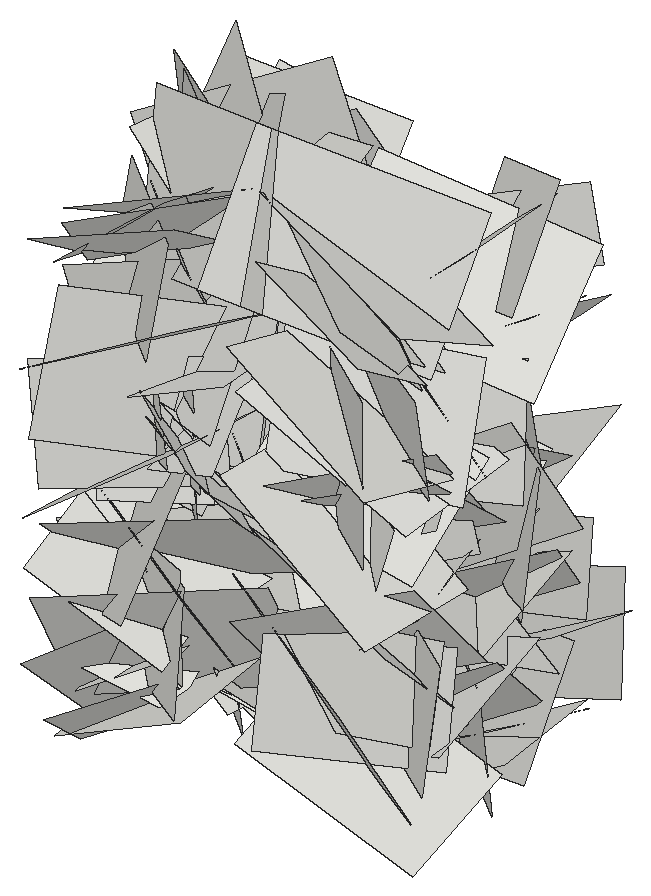
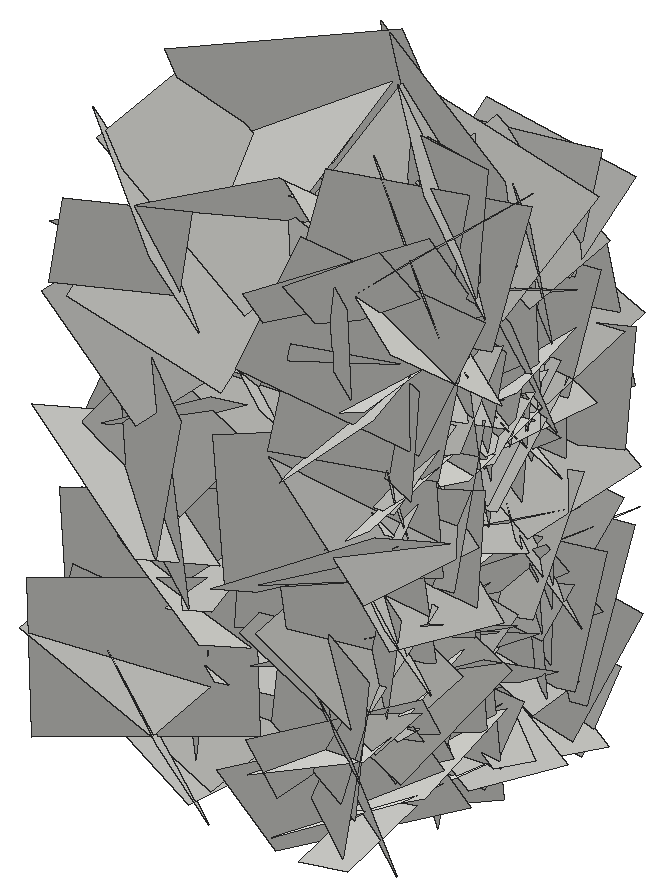
# SketchUp Ruby script. Lengths in inches.
U = 1.inch
M = Sketchup.active_model
def pt(a) = Geom::Point3d.new(a.map { |v| v * U })
def face(e, loops, mat)
  f = e.add_face(loops[0].map { |a| pt(a) })
  loops[1..].each { |l| e.add_face(l.map { |a| pt(a) }).erase! }
  f.material = f.back_material = mat if mat
  f
end
# faces: each face lists its corners as indices into pts; further lists are holes
def faces(e, pts, list, mat = nil) = list.each { |f| face(e, (f[0].is_a?(Array) ? f : [f]).map { |l| l.map { |i| pts[i] } }, mat) }
# xy, xz, yz: faces in a plane at the given z, y or x. An outline is a flat list of corners, or four numbers for a rectangle; further outlines are holes
def ring(l) = l.size == 4 ? [[l[0], l[1]], [l[2], l[1]], [l[2], l[3]], [l[0], l[3]]] : l.each_slice(2).to_a
def flat(e, list, mat, &to3) = list.each { |f| face(e, (f[0].is_a?(Array) ? f : [f]).map { |l| ring(l).map { |u, v| to3.(u, v) } }, mat) }
def xy(e, z, list, mat = nil) = flat(e, list, mat) { |x, y| [x, y, z] }
def xz(e, y, list, mat = nil) = flat(e, list, mat) { |x, z| [x, y, z] }
def yz(e, x, list, mat = nil) = flat(e, list, mat) { |y, z| [x, y, z] }
def lines(e, pts, list) = list.each { |a, b| e.add_line(pt(pts[a]), pt(pts[b])) }
# prism: a flat outline (further loops are holes) pulled along v
def prism(e, loops, v, mat = nil)
  f = face(e, loops, mat); d = Geom::Vector3d.new(v.map { |x| x * U })
  f.pushpull(f.normal.samedirection?(d) ? d.length : -d.length)
end
def box(e, o, s, mat = nil) = prism(e, [[o, [o[0] + s[0], o[1], o[2]], [o[0] + s[0], o[1] + s[1], o[2]], [o[0], o[1] + s[1], o[2]]]], [0, 0, s[2]], mat)
def at(x, y, z, deg = 0) = Geom::Transformation.translation(pt([x, y, z])) * Geom::Transformation.rotation(ORIGIN, Z_AXIS, deg.degrees)
def axes(o, x, y, z) = Geom::Transformation.new([*x, 0, *y, 0, *z, 0, *pt(o).to_a, 1])
def part(name) = M.definitions.add(name)
# library, detail: a bought-in or finely detailed component or shape, given as its bounding box
def library(name, o, s) = part(name).tap { |d| box(d.entities, o, s) }
def detail(e, o, s) = box(e.add_group.entities, o, s)
def put(e, d, t, mat = nil) = e.add_instance(d, t).tap { |i| i.material = mat if mat }
def group(e, t, mat = nil) = e.add_group.tap { |g| g.transformation = t; g.material = mat if mat }.entities
root = M.entities
c1 = part("Component\#6")
p = [[0.01,0,0],[0,3.24,4.54],[4.32,3.24,4.54],[4.33,0,0]]
faces(c1.entities,p,[[0,1,2,3]])
put(root,c1,axes([24.34,147.32,10.4375],[-0.06119,-0.47987,-0.75245],[-0.01649,-0.75336,0.48165],[0.94584,-0.04418,-0.04028]))
put(root,c1,axes([28.31,136.7,5.12],[-0.11008,0.58852,-0.4619],[0.03608,-0.46213,-0.59646],[-0.7922,-0.10282,0.03702]))
put(root,c1,axes([28.31,135.6875,17.375],[0.11773,0.10526,0.9962],[0.108,0.99592,-0.11659],[-1.05635,0.11356,0.09911]))
put(root,c1,axes([28.31,144.39,10.35],[0.12238,0.87118,-0.30871],[0.00416,-0.31157,-0.87778],[-0.97971,0.1075,-0.04229]))
put(root,c1,axes([24.34,139.94,18.75],[-0.02341,-0.9115,0.17831],[-0.09444,0.17962,0.90714],[0.97996,-0.00447,0.09169]))
put(root,c1,axes([28.31,141.47,13.3125],[0.15098,-0.93805,0.13539],[0.00567,0.13771,0.94846],[-1.00463,-0.1402,0.0257]))
put(root,c1,axes([28.31,143.17,8.1],[-0.04482,0.75985,0.07181],[-0.00358,0.07173,-0.76102],[-0.80902,-0.04241,-0.00061]))
put(root,c1,axes([28.31,139.62,7.21],[0.15609,-0.9187,-0.23757],[0.00588,-0.23958,0.92989],[-1.00583,-0.14396,-0.03143]))
put(root,c1,axes([24.34,145.65,3.28],[0.1646,0.60158,-0.34623],[0.0091,-0.35642,-0.61544],[0.73568,-0.13018,0.08507]))
put(root,c1,axes([28.31,141.35,5.69],[-0.05421,0.52298,-0.48745],[-0.04158,-0.49001,-0.52162],[-0.75668,-0.01054,0.06359]))
put(root,c1,axes([24.34,143.03,2.65],[-0.18528,-0.93043,-0.12384],[0.14778,-0.15031,0.9325],[0.98392,-0.15263,-0.16338]))
put(root,c1,axes([28.31,149.3125,5.88],[0.15882,-0.57412,-0.80425],[0.08368,-0.80389,0.58857],[-1.04409,-0.15176,-0.07517]))
put(root,c1,axes([28.31,141.5625,11.54],[0.13399,-0.80117,0.38482],[-0.02481,0.38556,0.81039],[-0.9418,-0.12414,0.0334]))
put(root,c1,axes([28.31,147.06,19.23],[0.16196,0.05609,-0.92604],[-0.00217,-0.93849,-0.05718],[-0.9834,0.01131,-0.15239]))
put(root,c1,axes([24.34,141.85,18.04],[-0.12661,-0.3078,1.12748],[-0.24587,1.11705,0.28038],[1.21422,0.1941,0.17434]))
put(root,c1,axes([28.31,142.57,12.97],[0.12959,-0.66136,0.5647],[-0.03976,0.56572,0.67067],[-0.92097,-0.11748,0.0505]))
put(root,c1,axes([28.31,147.56,10.64],[-0.00206,-0.13591,-0.77504],[0.03252,-0.77447,0.13573],[-0.83344,-0.02988,0.00721]))
put(root,c1,axes([24.34,143.95,11.7],[-0.02215,-0.88691,-0.38082],[-0.08723,-0.37788,0.88459],[1.0194,-0.05161,0.06742]))
put(root,c1,axes([24.34,144.05,16.5],[0.02895,-0.76847,-0.41691],[-0.01722,-0.41749,0.76847],[0.92657,0.01625,0.02731]))
put(root,c1,axes([28.31,143.33,2.25],[-0.06381,-0.71847,0.0034],[0.02834,0.00117,0.7205],[-0.76106,0.06028,0.02655]))
put(root,c1,axes([24.34,147.01,9.44],[-0.18802,-1.10018,-0.17062],[-0.06994,-0.16208,1.11371],[1.17806,-0.18521,0.03889]))
put(root,c1,axes([24.34,143.66,16.18],[0.1105,0.58717,-0.52568],[0.01323,-0.53143,-0.59111],[0.83529,-0.06926,0.0789]))
put(root,c1,axes([24.34,145.52,18.22],[-0.02537,0.1253,-0.85934],[0.08829,-0.85537,-0.12704],[0.91628,0.08589,-0.01155]))
put(root,c1,axes([28.31,146.8125,4.55],[0.17148,-0.83232,0.10491],[-0.08015,0.09194,0.84603],[-0.88562,-0.16948,-0.05625]))
put(root,c1,axes([24.34,139.77,3.95],[0.11908,-0.78329,-0.0515],[0.03618,-0.0471,0.79084],[0.83129,0.11425,-0.02704]))
put(root,c1,axes([24.34,143.76,15.19],[0.09057,0.86782,-0.29614],[-0.1091,-0.28647,-0.86917],[0.96584,-0.11373,-0.07041]))
put(root,c1,axes([28.31,138.58,20.36],[0.30182,0.3301,1.08442],[0.18064,1.09293,-0.37743],[-1.1879,0.25007,0.21813]))
put(root,c1,axes([24.34,142.07,24.73],[-0.13514,0.30002,-0.93652],[0.09595,-0.93677,-0.31242],[1.03799,0.12565,-0.09305]))
put(root,c1,axes([28.31,143.53,7.33],[0.11895,-0.88372,0.009],[0.0734,0.01784,0.88799],[-0.93392,-0.11115,0.07094]))
put(root,c1,axes([24.34,139.41,15.5],[0.07329,-0.02436,0.98546],[-0.16551,0.97513,0.03506],[1.03171,0.15816,-0.06438]))
put(root,c1,axes([28.31,142.73,15.75],[0.26089,1.021,-0.12695],[0.10549,-0.15355,-1.04195],[-1.08548,0.23047,-0.13178]))
put(root,c1,axes([28.31,136.74,12.93],[-0.11437,0.04247,0.59628],[-0.02624,0.60507,-0.04758],[-0.63311,-0.03275,-0.10574]))
put(root,c1,axes([24.34,145.52,15.88],[-0.20612,-0.51117,0.96001],[0.04532,0.97089,0.52562],[1.15198,-0.12966,0.1511]))
put(root,c1,axes([28.31,139.35,17.19],[-0.06054,-0.33637,0.61942],[0.0607,0.61718,0.34043],[-0.74468,0.07766,-0.02261]))
put(root,c1,axes([28.31,143.63,3.63],[-0.04495,-0.13338,0.65571],[-0.00407,0.65706,0.13341],[-0.70927,0.00468,-0.04233]))
put(root,c1,axes([28.31,140.67,1.375],[-0.09858,-0.02009,0.69473],[0.09996,0.69407,0.03269],[-0.72991,0.09776,-0.08935]))
put(root,c1,axes([24.34,137.55,18.4],[-0.05522,0.7917,0.38208],[0.20111,0.38385,-0.76951],[0.90986,-0.0368,0.19328]))
put(root,c1,axes([28.31,141.96,13.08],[-0.07799,-0.57044,-0.33182],[0.05167,-0.33766,0.56968],[-0.69762,0.03877,0.07929]))
put(root,c1,axes([24.34,146.4375,4.35],[-0.18242,-1.06895,0.55133],[-0.10581,0.56772,1.06956],[1.27052,-0.1062,0.16823]))
put(root,c1,axes([24.34,139.48,6.78],[0.1397,0.74364,0.31774],[0.04551,0.31504,-0.75514],[0.85599,-0.13812,-0.01171]))
put(root,c1,axes([28.31,147.44,21.48],[-0.11936,-0.32986,-0.48912],[0.02265,-0.49991,0.33221],[-0.62494,0.04489,0.10546]))
put(root,c1,axes([28.31,139.2,5.38],[0.02645,-0.5119,-0.36479],[-0.13209,-0.36186,0.49927],[-0.65307,0.05245,-0.11575]))
put(root,c1,axes([24.34,137.79,2.1],[-0.03475,-0.78477,0.75119],[-0.11687,0.75006,0.77877],[1.14558,0.05272,0.10224]))
put(root,c1,axes([28.31,141.75,2.2],[-0.07408,-0.19814,0.56205],[-0.01701,0.56632,0.19765],[-0.63148,0.00798,-0.07126]))
put(root,c1,axes([24.34,135.11,11.54],[-0.10699,0.00448,1.06975],[0.01257,1.07444,-0.00338],[1.13388,-0.01149,0.10098]))
put(root,c1,axes([28.31,139.97,19.34],[0.20036,-0.21311,0.82685],[0.01235,0.84743,0.21575],[-0.90502,-0.03562,0.186]))
put(root,c1,axes([24.34,145.41,21.68],[0.17174,-0.50133,-0.77339],[-0.12403,-0.79008,0.48764],[0.96905,-0.01227,0.19948]))
put(root,c1,axes([28.31,141.82,12.65],[-0.04235,0.31596,0.66399],[0.14644,0.65635,-0.30401],[-0.76557,0.10807,-0.09488]))
put(root,c1,axes([24.34,136.25,6.15],[0.02753,0.62765,0.83331],[-0.11118,0.83092,-0.62258],[1.10023,0.06826,-0.08377]))
put(root,c1,axes([24.34,142.09,4.39],[0.13266,-0.06807,0.83796],[0.05074,0.84639,0.06161],[0.88972,-0.03812,-0.12846]))
put(root,c1,axes([24.34,149.05,6.52],[-0.16475,-0.3536,-1.09271],[-0.00842,-1.10231,0.35784],[1.21738,-0.05548,-0.1454]))
put(root,c1,axes([28.31,138.56,10.4375],[0.05239,0.37979,0.51244],[-0.10197,0.51253,-0.37059],[-0.66837,-0.04842,0.0967]))
put(root,c1,axes([24.34,141.11,17.69],[0.01651,0.23078,-0.87547],[0.12637,-0.8685,-0.22682],[0.95135,0.11136,0.04532]))
put(root,c1,axes([24.34,140.66,10.67],[-0.05387,-0.70807,-1.02445],[-0.25854,-0.99979,0.70312],[1.29449,-0.22915,0.09779]))
put(root,c1,axes([28.31,145.32,5.58],[-0.01721,-0.24816,-0.73855],[0.187,-0.7207,0.23828],[-0.80443,-0.16223,0.07119]))
put(root,c1,axes([24.34,139.9,15.42],[0.08068,-0.00169,-0.87701],[0.08263,-0.87681,0.00845],[0.92595,0.07839,0.07566]))
put(root,c1,axes([28.31,139.99,14.29],[-0.01199,-0.16574,0.68191],[0.09091,0.67656,0.16586],[-0.73829,0.086,0.00935]))
put(root,c1,axes([28.31,147.58,14.43],[0.15626,-0.88067,0.15465],[0.14549,0.17716,0.87807],[-0.93656,-0.11942,0.1622]))
put(root,c1,axes([28.31,138.3,10.21],[0.07821,-0.14386,0.79141],[0.12147,0.78851,0.13265],[-0.84394,0.10016,0.09244]))
put(root,c1,axes([24.34,142.2,15.72],[-0.2001,0.61396,-1.10583],[-0.10306,-1.12181,-0.60624],[1.33676,0.00542,-0.21228]))
put(root,c1,axes([24.34,141.25,1.55],[0.11713,-0.0063,1.0149],[-0.13715,1.01248,0.02037],[1.06704,0.13083,-0.10878]))
put(root,c1,axes([24.34,144.34,6.82],[-0.01542,0.93301,-0.17325],[0.14993,-0.1692,-0.92309],[0.99466,0.03997,0.13646]))
put(root,c1,axes([24.34,137.99,14.66],[-0.08461,-0.27233,0.9902],[0.1352,0.98287,0.28059],[1.08015,-0.14435,0.04245]))
put(root,c1,axes([24.34,142.29,19.52],[0.02505,0.60517,0.90894],[-0.1077,0.90642,-0.60085],[1.15246,0.07156,-0.07591]))
put(root,c1,axes([24.34,144.58,9.97],[0.16827,0.58944,-0.69808],[-0.0398,-0.70373,-0.60275],[0.96765,-0.13145,0.0966]))
put(root,c1,axes([28.31,139.8125,20.98],[-0.02151,0.52563,-0.34386],[0.05265,-0.34162,-0.52514],[-0.66372,-0.04413,-0.03051]))
put(root,c1,axes([28.31,142.6,14.22],[0.18899,-0.6396,-0.42028],[-0.00285,-0.43205,0.65638],[-0.81124,-0.14749,-0.10022]))
put(root,c1,axes([28.31,145.36,10.15],[0.14636,-0.64891,0.3527],[0.01811,0.36152,0.65845],[-0.78267,-0.11298,0.08119]))
put(root,c1,axes([28.31,145.42,18.19],[0.07853,-0.05807,0.70782],[0.06912,0.70921,0.05136],[-0.74963,0.05931,0.07889]))
put(root,c1,axes([24.34,146.45,10.34],[0.10559,0.05407,-0.92917],[0.0532,-0.93343,-0.04894],[0.98516,0.04461,0.10223]))
put(root,c1,axes([28.31,141.95,12.73],[0.09992,0.55515,0.3498],[-0.02862,0.35638,-0.5583],[-0.69495,0.06514,0.07329]))
put(root,c1,axes([24.34,137.63,3.85],[-0.23328,-0.07655,1.22947],[0.08564,1.24535,0.092],[1.30295,-0.09556,0.21407]))
put(root,c1,axes([24.34,137.89,18.97],[0.02244,-0.79516,0.48934],[0.22215,0.48102,0.77258],[0.96443,-0.0923,-0.18934]))
put(root,c1,axes([28.31,139.18,13.74],[0.11062,-0.13563,-0.63299],[-0.03095,-0.6415,0.13263],[-0.6855,0.00708,-0.10814]))
put(root,c1,axes([24.34,141.92,3.18],[0.02887,1.0089,0.10446],[0.06921,0.10254,-1.00735],[1.07292,-0.03376,0.06217]))
put(root,c1,axes([24.34,138.34,13.4],[0.1901,0.66514,0.65147],[-0.02496,0.66648,-0.67398],[0.98658,-0.1113,-0.14258]))
put(root,c1,axes([24.34,138.76,9.15],[0.08107,-0.07376,-0.93469],[0.12107,-0.93007,0.08274],[0.98644,0.12021,0.06666]))
put(root,c1,axes([24.34,139.52,8.83],[0.01584,-0.12995,-1.07448],[0.00128,-1.07458,0.12998],[1.14724,0.003,0.01469]))
put(root,c1,axes([24.34,137.41,10.49],[0.17918,0.96529,0.20208],[-0.06958,0.21558,-0.97489],[1.04307,-0.15144,-0.09975]))
put(root,c1,axes([24.34,141.07,4.77],[-0.0925,1.07709,-0.24358],[0.13853,-0.23255,-1.07513],[1.16232,0.11343,0.10875]))
put(root,c1,axes([24.34,143.54,11.83],[-0.01207,0.98557,0.48784],[0.03058,0.48797,-0.98515],[1.16528,-0.0026,0.03091]))
put(root,c1,axes([28.31,142.82,6.12],[-0.04161,-0.60559,-0.03198],[0.13563,-0.03959,0.59276],[-0.62835,0.03156,0.13006]))
put(root,c1,axes([24.34,142.72,8.07],[-0.13823,0.05764,1.30603],[-0.0986,1.30878,-0.06705],[1.38223,0.09912,0.12583]))
put(root,c1,axes([24.34,138.64,15.1],[-0.05154,1.07135,-0.23626],[0.10153,-0.23144,-1.06922],[1.15847,0.06794,0.08319]))
put(root,c1,axes([24.34,138.49,4.97],[-0.13436,1.04009,0.6085],[0.04809,0.61554,-1.04268],[1.27641,0.08629,0.10334]))
put(root,c1,axes([28.31,137.29,3.46],[0.14224,0.61257,0.15159],[-0.04066,0.16261,-0.62315],[-0.66768,0.1206,0.07024]))
put(root,c1,axes([24.34,137.21,11.6875],[-0.11385,0.72886,-0.88593],[0.14818,-0.87485,-0.7367],[1.20699,0.17615,0.00688]))
put(root,c1,axes([24.34,143.17,19.13],[0.20193,0.9279,-0.28366],[0.04691,-0.29708,-0.94209],[1.02744,-0.16881,0.09877]))
put(root,c1,axes([24.34,142.88,1.98],[0.0351,0.64216,0.95117],[0.00533,0.95147,-0.64254],[1.21649,-0.02269,-0.02463]))
put(root,c1,axes([24.34,137.64,18.89],[0.26376,-0.64139,0.69016],[0.02251,0.71746,0.65911],[0.99845,0.15326,-0.19718]))
put(root,c1,axes([24.34,140.93,18.6875],[-0.10901,-0.41314,-1.06231],[0.28274,-1.04573,0.38087],[1.17466,0.21337,-0.19026]))
put(root,c1,axes([24.34,141.75,2.91],[-0.11729,-1.19784,-0.30033],[0.11289,-0.30967,1.19584],[1.30414,-0.08092,-0.13053]))
put(root,c1,axes([24.34,143.08,17.68],[-0.06532,-0.13436,-1.17102],[0.13166,-1.16683,0.12734],[1.24247,0.11658,-0.07506]))
put(root,c1,axes([24.34,140.04,10.48],[-0.03722,-1.27767,0.05021],[-0.04996,0.05148,1.27723],[1.35446,-0.03321,0.04849]))
put(root,c1,axes([24.34,140.59,7.56],[-0.03383,1.06332,0.50099],[0.10932,0.50178,-1.05842],[1.24115,-0.01522,0.10688]))
put(root,c1,axes([24.34,137.94,15.45],[-0.03401,0.89045,-0.73196],[0.17038,-0.72163,-0.88493],[1.2099,0.12665,0.10405]))
put(root,c1,axes([24.34,146.96,20.2],[-0.19126,-1.0536,-0.82739],[0.10265,-0.84293,1.05228],[1.41631,-0.08119,-0.188]))
put(root,c1,axes([24.34,139.77,22.87],[0.12093,1.26112,-0.05281],[-0.18505,-0.03675,-1.25475],[1.32509,-0.12022,-0.17041]))
put(root,c1,axes([24.34,139.44,14.86],[-0.04621,-1.16691,0.31838],[0.12643,0.31289,1.16311],[1.27589,-0.07327,-0.10372]))
put(root,c1,axes([24.34,141.48,7.17],[0.20337,0.82379,-0.77749],[-0.08888,-0.77608,-0.84298],[1.19742,-0.19752,0.06948]))
put(root,c1,axes([24.34,138.37,16.22],[0.07456,0.76169,-0.90937],[0.0504,-0.91204,-0.76025],[1.25638,-0.00862,0.08446]))
put(root,c1,axes([24.34,148.05,8.79],[0.07068,0.0827,-1.14811],[0.1221,-1.14474,-0.07576],[1.21402,0.11031,0.07447]))
put(root,c1,axes([24.34,144.3,10.94],[0.16969,-0.07735,1.18237],[-0.06112,1.19119,0.08573],[1.2545,0.0685,-0.15576]))
put(root,c1,axes([24.34,144.73,5.33],[0.04426,-1.02294,0.56209],[0.16257,0.56238,1.01208],[1.2265,-0.03763,-0.15444]))
put(root,c1,axes([24.34,141.11,14.91],[0.10517,-0.78429,-0.79452],[0.18451,-0.77703,0.78876],[1.16892,0.19321,-0.05302]))
put(root,c1,axes([24.34,134.59,13.6],[0.14779,0.17555,1.29716],[-0.16453,1.29751,-0.15892],[1.37773,0.13612,-0.15813]))
put(root,c1,axes([24.34,148.13,7.79],[0.13698,0.11741,-1.23467],[-0.05668,-1.23967,-0.12348],[1.31343,-0.06574,0.12344]))
put(root,c1,axes([24.34,139.3125,6.46],[-0.05297,-0.89114,0.82127],[0.332,0.78454,0.87035],[1.24093,-0.24794,-0.1978]))
put(root,c1,axes([24.34,142.16,14.375],[-0.02255,-1.26636,-0.09652],[0.2141,-0.09868,1.25016],[1.3291,-0.00559,-0.20302]))
put(root,c1,axes([24.34,141.32,18.93],[-0.00931,-1.12138,0.55372],[0.26786,0.54072,1.09906],[1.29833,-0.1196,-0.22278]))
put(root,c1,axes([24.34,140.96,14.21],[0.1647,-0.56811,1.02456],[0.16232,1.03452,0.5504],[1.23116,-0.0604,-0.20963]))
put(root,c1,axes([24.34,137.06,3.09],[0.11239,-0.69918,1.17187],[0.18512,1.17269,0.68387],[1.43458,-0.09655,-0.18006]))
put(root,c1,axes([24.34,141.18,23.91],[0.20239,-0.45291,-1.29893],[0.24414,-1.28235,0.48098],[1.43758,0.28153,0.10118]))
put(root,c1,axes([38.11,141.18,23.91],[-0.20239,-0.45291,-1.29893],[-0.24414,-1.28235,0.48098],[-1.43758,0.28153,0.10118]))
put(root,c1,axes([38.11,137.06,3.09],[-0.11239,-0.69918,1.17187],[-0.18512,1.17269,0.68387],[-1.43458,-0.09655,-0.18006]))
put(root,c1,axes([38.11,140.96,14.21],[-0.1647,-0.56811,1.02456],[-0.16232,1.03452,0.5504],[-1.23116,-0.0604,-0.20963]))
put(root,c1,axes([38.11,141.32,18.93],[0.00931,-1.12138,0.55372],[-0.26786,0.54072,1.09906],[-1.29833,-0.1196,-0.22278]))
put(root,c1,axes([38.11,142.16,14.375],[0.02255,-1.26636,-0.09652],[-0.2141,-0.09868,1.25016],[-1.3291,-0.00559,-0.20302]))
put(root,c1,axes([38.11,139.3125,6.46],[0.05297,-0.89114,0.82127],[-0.332,0.78454,0.87035],[-1.24093,-0.24794,-0.1978]))
put(root,c1,axes([38.11,148.13,7.79],[-0.13698,0.11741,-1.23467],[0.05668,-1.23967,-0.12348],[-1.31343,-0.06574,0.12344]))
put(root,c1,axes([38.11,134.59,13.6],[-0.14779,0.17555,1.29716],[0.16453,1.29751,-0.15892],[-1.37773,0.13612,-0.15813]))
put(root,c1,axes([38.11,141.11,14.91],[-0.10517,-0.78429,-0.79452],[-0.18451,-0.77703,0.78876],[-1.16892,0.19321,-0.05302]))
put(root,c1,axes([38.11,144.73,5.33],[-0.04426,-1.02294,0.56209],[-0.16257,0.56238,1.01208],[-1.2265,-0.03763,-0.15444]))
put(root,c1,axes([38.11,144.3,10.94],[-0.16969,-0.07735,1.18237],[0.06112,1.19119,0.08573],[-1.2545,0.0685,-0.15576]))
put(root,c1,axes([38.11,138.37,16.22],[-0.07456,0.76169,-0.90937],[-0.0504,-0.91204,-0.76025],[-1.25638,-0.00862,0.08446]))
put(root,c1,axes([38.11,141.48,7.17],[-0.20337,0.82379,-0.77749],[0.08888,-0.77608,-0.84298],[-1.19742,-0.19752,0.06948]))
put(root,c1,axes([38.11,139.44,14.86],[0.04621,-1.16691,0.31838],[-0.12643,0.31289,1.16311],[-1.27589,-0.07327,-0.10372]))
put(root,c1,axes([38.11,139.77,22.87],[-0.12093,1.26112,-0.05281],[0.18505,-0.03675,-1.25475],[-1.32509,-0.12022,-0.17041]))
put(root,c1,axes([38.11,146.96,20.2],[0.19126,-1.0536,-0.82739],[-0.10265,-0.84293,1.05228],[-1.41631,-0.08119,-0.188]))
put(root,c1,axes([38.11,137.94,15.45],[0.03401,0.89045,-0.73196],[-0.17038,-0.72163,-0.88493],[-1.2099,0.12665,0.10405]))
put(root,c1,axes([38.11,140.59,7.56],[0.03383,1.06332,0.50099],[-0.10932,0.50178,-1.05842],[-1.24115,-0.01522,0.10688]))
put(root,c1,axes([38.11,140.04,10.48],[0.03722,-1.27767,0.05021],[0.04996,0.05148,1.27723],[-1.35446,-0.03321,0.04849]))
put(root,c1,axes([38.11,143.08,17.68],[0.06532,-0.13436,-1.17102],[-0.13166,-1.16683,0.12734],[-1.24247,0.11658,-0.07506]))
put(root,c1,axes([38.11,141.75,2.91],[0.11729,-1.19784,-0.30033],[-0.11289,-0.30967,1.19584],[-1.30414,-0.08092,-0.13053]))
put(root,c1,axes([38.11,140.93,18.6875],[0.10901,-0.41314,-1.06231],[-0.28274,-1.04573,0.38087],[-1.17466,0.21337,-0.19026]))
put(root,c1,axes([38.11,137.64,18.89],[-0.26376,-0.64139,0.69016],[-0.02251,0.71746,0.65911],[-0.99845,0.15326,-0.19718]))
put(root,c1,axes([38.11,142.88,1.98],[-0.0351,0.64216,0.95117],[-0.00533,0.95147,-0.64254],[-1.21649,-0.02269,-0.02463]))
put(root,c1,axes([38.11,143.17,19.13],[-0.20193,0.9279,-0.28366],[-0.04691,-0.29708,-0.94209],[-1.02744,-0.16881,0.09877]))
put(root,c1,axes([38.11,137.21,11.6875],[0.11385,0.72886,-0.88593],[-0.14818,-0.87485,-0.7367],[-1.20699,0.17615,0.00688]))
put(root,c1,axes([34.14,137.29,3.46],[-0.14224,0.61257,0.15159],[0.04066,0.16261,-0.62315],[0.66768,0.1206,0.07024]))
put(root,c1,axes([38.11,138.49,4.97],[0.13436,1.04009,0.6085],[-0.04809,0.61554,-1.04268],[-1.27641,0.08629,0.10334]))
put(root,c1,axes([38.11,138.64,15.1],[0.05154,1.07135,-0.23626],[-0.10153,-0.23144,-1.06922],[-1.15847,0.06794,0.08319]))
put(root,c1,axes([38.11,142.72,8.07],[0.13823,0.05764,1.30603],[0.0986,1.30878,-0.06705],[-1.38223,0.09912,0.12583]))
put(root,c1,axes([34.14,142.82,6.12],[0.04161,-0.60559,-0.03198],[-0.13563,-0.03959,0.59276],[0.62835,0.03156,0.13006]))
put(root,c1,axes([38.11,143.54,11.83],[0.01207,0.98557,0.48784],[-0.03058,0.48797,-0.98515],[-1.16528,-0.0026,0.03091]))
put(root,c1,axes([38.11,141.07,4.77],[0.0925,1.07709,-0.24358],[-0.13853,-0.23255,-1.07513],[-1.16232,0.11343,0.10875]))
put(root,c1,axes([38.11,137.41,10.49],[-0.17918,0.96529,0.20208],[0.06958,0.21558,-0.97489],[-1.04307,-0.15144,-0.09975]))
put(root,c1,axes([38.11,139.52,8.83],[-0.01584,-0.12995,-1.07448],[-0.00128,-1.07458,0.12998],[-1.14724,0.003,0.01469]))
put(root,c1,axes([38.11,138.76,9.15],[-0.08107,-0.07376,-0.93469],[-0.12107,-0.93007,0.08274],[-0.98644,0.12021,0.06666]))
put(root,c1,axes([38.11,138.34,13.4],[-0.1901,0.66514,0.65147],[0.02496,0.66648,-0.67398],[-0.98658,-0.1113,-0.14258]))
put(root,c1,axes([38.11,141.92,3.18],[-0.02887,1.0089,0.10446],[-0.06921,0.10254,-1.00735],[-1.07292,-0.03376,0.06217]))
put(root,c1,axes([34.14,139.18,13.74],[-0.11062,-0.13563,-0.63299],[0.03095,-0.6415,0.13263],[0.6855,0.00708,-0.10814]))
put(root,c1,axes([38.11,137.89,18.97],[-0.02244,-0.79516,0.48934],[-0.22215,0.48102,0.77258],[-0.96443,-0.0923,-0.18934]))
put(root,c1,axes([38.11,137.63,3.85],[0.23328,-0.07655,1.22947],[-0.08564,1.24535,0.092],[-1.30295,-0.09556,0.21407]))
put(root,c1,axes([34.14,141.95,12.73],[-0.09992,0.55515,0.3498],[0.02862,0.35638,-0.5583],[0.69495,0.06514,0.07329]))
put(root,c1,axes([38.11,146.45,10.34],[-0.10559,0.05407,-0.92917],[-0.0532,-0.93343,-0.04894],[-0.98516,0.04461,0.10223]))
put(root,c1,axes([34.14,145.42,18.19],[-0.07853,-0.05807,0.70782],[-0.06912,0.70921,0.05136],[0.74963,0.05931,0.07889]))
put(root,c1,axes([34.14,145.36,10.15],[-0.14636,-0.64891,0.3527],[-0.01811,0.36152,0.65845],[0.78267,-0.11298,0.08119]))
put(root,c1,axes([34.14,142.6,14.22],[-0.18899,-0.6396,-0.42028],[0.00285,-0.43205,0.65638],[0.81124,-0.14749,-0.10022]))
put(root,c1,axes([34.14,139.8125,20.98],[0.02151,0.52563,-0.34386],[-0.05265,-0.34162,-0.52514],[0.66372,-0.04413,-0.03051]))
put(root,c1,axes([38.11,144.58,9.97],[-0.16827,0.58944,-0.69808],[0.0398,-0.70373,-0.60275],[-0.96765,-0.13145,0.0966]))
put(root,c1,axes([38.11,142.29,19.52],[-0.02505,0.60517,0.90894],[0.1077,0.90642,-0.60085],[-1.15246,0.07156,-0.07591]))
put(root,c1,axes([38.11,137.99,14.66],[0.08461,-0.27233,0.9902],[-0.1352,0.98287,0.28059],[-1.08015,-0.14435,0.04245]))
put(root,c1,axes([38.11,144.34,6.82],[0.01542,0.93301,-0.17325],[-0.14993,-0.1692,-0.92309],[-0.99466,0.03997,0.13646]))
put(root,c1,axes([38.11,141.25,1.55],[-0.11713,-0.0063,1.0149],[0.13715,1.01248,0.02037],[-1.06704,0.13083,-0.10878]))
put(root,c1,axes([38.11,142.2,15.72],[0.2001,0.61396,-1.10583],[0.10306,-1.12181,-0.60624],[-1.33676,0.00542,-0.21228]))
put(root,c1,axes([34.14,138.3,10.21],[-0.07821,-0.14386,0.79141],[-0.12147,0.78851,0.13265],[0.84394,0.10016,0.09244]))
put(root,c1,axes([34.14,147.58,14.43],[-0.15626,-0.88067,0.15465],[-0.14549,0.17716,0.87807],[0.93656,-0.11942,0.1622]))
